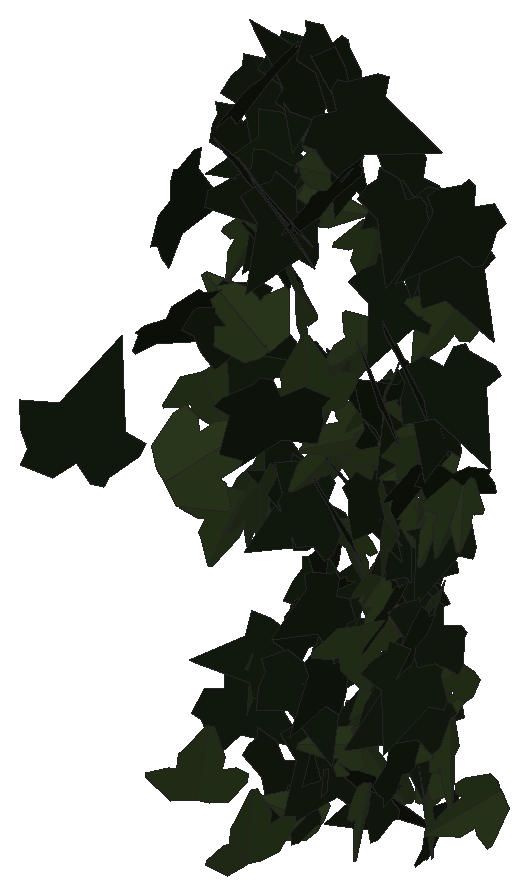
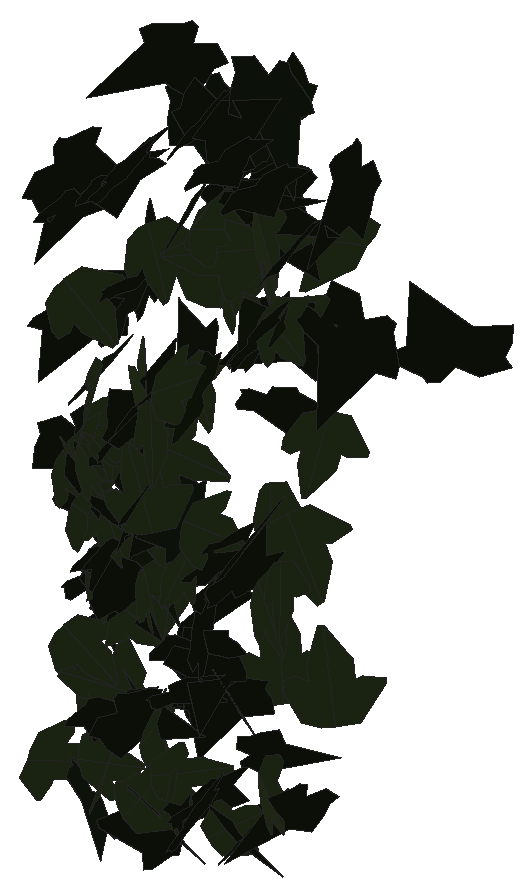
# SketchUp Ruby script. Lengths in inches.
U = 1.inch
M = Sketchup.active_model
def pt(a) = Geom::Point3d.new(a.map { |v| v * U })
def face(e, loops, mat)
  f = e.add_face(loops[0].map { |a| pt(a) })
  loops[1..].each { |l| e.add_face(l.map { |a| pt(a) }).erase! }
  f.material = f.back_material = mat if mat
  f
end
# faces: each face lists its corners as indices into pts; further lists are holes
def faces(e, pts, list, mat = nil) = list.each { |f| face(e, (f[0].is_a?(Array) ? f : [f]).map { |l| l.map { |i| pts[i] } }, mat) }
# xy, xz, yz: faces in a plane at the given z, y or x. An outline is a flat list of corners, or four numbers for a rectangle; further outlines are holes
def ring(l) = l.size == 4 ? [[l[0], l[1]], [l[2], l[1]], [l[2], l[3]], [l[0], l[3]]] : l.each_slice(2).to_a
def flat(e, list, mat, &to3) = list.each { |f| face(e, (f[0].is_a?(Array) ? f : [f]).map { |l| ring(l).map { |u, v| to3.(u, v) } }, mat) }
def xy(e, z, list, mat = nil) = flat(e, list, mat) { |x, y| [x, y, z] }
def xz(e, y, list, mat = nil) = flat(e, list, mat) { |x, z| [x, y, z] }
def yz(e, x, list, mat = nil) = flat(e, list, mat) { |y, z| [x, y, z] }
def lines(e, pts, list) = list.each { |a, b| e.add_line(pt(pts[a]), pt(pts[b])) }
# prism: a flat outline (further loops are holes) pulled along v
def prism(e, loops, v, mat = nil)
  f = face(e, loops, mat); d = Geom::Vector3d.new(v.map { |x| x * U })
  f.pushpull(f.normal.samedirection?(d) ? d.length : -d.length)
end
def box(e, o, s, mat = nil) = prism(e, [[o, [o[0] + s[0], o[1], o[2]], [o[0] + s[0], o[1] + s[1], o[2]], [o[0], o[1] + s[1], o[2]]]], [0, 0, s[2]], mat)
def at(x, y, z, deg = 0) = Geom::Transformation.translation(pt([x, y, z])) * Geom::Transformation.rotation(ORIGIN, Z_AXIS, deg.degrees)
def axes(o, x, y, z) = Geom::Transformation.new([*x, 0, *y, 0, *z, 0, *pt(o).to_a, 1])
def part(name) = M.definitions.add(name)
# library, detail: a bought-in or finely detailed component or shape, given as its bounding box
def library(name, o, s) = part(name).tap { |d| box(d.entities, o, s) }
def detail(e, o, s) = box(e.add_group.entities, o, s)
def put(e, d, t, mat = nil) = e.add_instance(d, t).tap { |i| i.material = mat if mat }
def group(e, t, mat = nil) = e.add_group.tap { |g| g.transformation = t; g.material = mat if mat }.entities
root = M.entities
M.materials.add("efeu1").color = [18, 25, 13]
M.materials.add("efeu2").color = [43, 57, 29]
c1 = part("ivyleaf_10")
p = [[0,0.5,-0.03],[-0.0625,2.02,-0.43],[-0.19,2.01,-0.46],[-0.54,1.05,-0.29],[-0.52,0.625,-0.18],[-0.83,0.76,-0.28],
  [-1.16,0.64,-0.33],[-1.15,0.33,-0.24],[-0.77,-0.39,0.02],[-0.3,-0.51,0.16],[0.04,-0.48,0.23],[-0.02,2.01,-0.4375],
  [-0.06,2.01,-0.43],[0.04,-0.49,0.23],[0.67,-0.49,0.14],[1.38,0.36,-0.2],[1.375,0.51,-0.24],[0.81,0.65,-0.19],
  [0.62,0.59,-0.15],[0.6,1.09,-0.28],[0.5,1.23,-0.31]]
faces(c1.entities,p,[[0,1,2,3,4,5,6,7,8,9,10],[11,12,0,13,14,15,16,17,18,19,20]],"efeu2")
c2 = part("ivyleaf_9")
p = [[1.54,2.16,1.25],[1.36,2.04,1.19],[-0.21,0.99,0.68],[-0.71,1.11,0.82],[-0.85,0.86,0.67],[-0.8,0.17,0.21],
  [-0.9,-0.01,0.1],[-0.67,-0.16,-0.02],[-0.08,-0.08,-0.05],[-0.03,-0.6,-0.4],[0.65,-0.88,-0.66],[0.83,-0.6,-0.49],
  [1.29,-0.42,-0.43],[1.8125,-0.07,-0.26],[1.21,0.44,0.15]]
faces(c2.entities,p,[[0,1,2,3,4,5,6,7,8,9,10,11,12,13,14]],"efeu1")
put(root,c1,axes([531.67,124.5,197.65],[0.51111,0.17788,-1.07304],[0.73605,0.81633,0.48592],[0.8008,-0.86385,0.23824]))
put(root,c2,axes([527.39,125.43,196.0625],[-0.81368,-0.12856,0.81863],[0.8051,0.14899,0.82363],[-0.19619,1.14456,-0.01526]))
put(root,c2,axes([533.48,126.2,199.56],[0.07548,0.58872,-0.9233],[-0.13977,-0.91274,-0.59341],[-1.08606,0.15838,0.0122]))
put(root,c1,axes([532.22,126.64,185.43],[-0.3475,-1.0008,-0.16593],[-0.05095,-0.15796,1.0594],[-1.01318,0.3512,0.00364]))
put(root,c1,axes([529.72,127.6,186.04],[-0.77998,-0.69849,0.07567],[0.05931,0.04719,1.04701],[-0.70006,0.78222,0.0044]))
put(root,c2,axes([533.3,128.66,195.09],[0.69791,-0.24708,-0.62973],[0.62363,-0.11557,0.73649],[-0.2621,-0.93289,0.07555]))
put(root,c1,axes([532.47,128.77,198.07],[-0.705,-0.83813,-0.16697],[-0.1081,-0.12726,1.09521],[-0.84774,0.71324,-0.00079]))
put(root,c2,axes([530.03,129.12,203.81],[0.57878,-0.62248,0.69314],[0.53625,-0.44467,-0.84712],[0.76181,0.78593,0.06969]))
put(root,c2,axes([531.34,129.53,202.91],[-0.25695,-0.80421,0.44674],[-0.15046,-0.42086,-0.84415],[0.90758,-0.29745,-0.01347]))
put(root,c2,axes([530.54,129.21,203.48],[0.56679,-0.62146,0.50238],[0.33472,-0.37466,-0.8411],[0.72565,0.65824,-0.00442]))
put(root,c2,axes([528.23,128.375,202.71],[0.03539,0.10523,-1.08229],[-0.74277,0.79321,0.05283],[0.79418,0.73717,0.09764]))
put(root,c2,axes([533.78,130.09,198.03],[-0.08215,-0.25819,0.96773],[0.28098,-0.93793,-0.22639],[0.96136,0.25207,0.14886]))
put(root,c2,axes([532.42,129.54,203.96],[-0.33089,0.95802,-0.29231],[0.08395,-0.28024,-1.01348],[-0.99809,-0.34117,0.01166]))
put(root,c2,axes([527.61,129,198.71],[0.38203,0.98395,0.23303],[0.0845,0.21717,-1.05551],[-1.00763,0.39127,-0.00016]))
put(root,c2,axes([534.6875,130.42,190.02],[-0.37882,-0.71589,0.04601],[-0.01389,-0.0447,-0.80989],[0.71723,-0.37898,0.00862]))
put(root,c1,axes([529.51,130.28,198.34],[0.62928,0.4348,0.68302],[-0.59696,-0.33525,0.76342],[0.54699,-0.86609,0.04739]))
put(root,c1,axes([528.6,130.57,192.83],[-0.53811,-0.78375,0.34572],[-0.18084,-0.29513,-0.95054],[0.8373,-0.56743,0.01689]))
put(root,c2,axes([528.52,130.05,198.85],[0.10065,-0.13279,-0.94088],[0.38967,0.86869,-0.08091],[0.86663,-0.37518,0.14566]))
put(root,c1,axes([532.88,130.43,190.41],[-0.58926,-0.74693,-0.07449],[0.03867,0.06436,-0.95133],[0.74963,-0.59045,-0.00947]))
put(root,c2,axes([534.42,131.3,188.79],[-0.54804,-0.56212,0.5967],[-0.32904,-0.50657,-0.77943],[0.75084,-0.63229,0.09397]))
put(root,c1,axes([527.66,130.48,196.2],[-0.5787,-0.66826,-0.24815],[0.18638,0.16666,-0.88348],[0.68805,-0.6072,0.03061]))
put(root,c1,axes([532.57,130.9,185.26],[0.55846,-0.42346,0.37129],[0.28299,-0.24108,-0.70061],[0.48692,0.62579,-0.01865]))
put(root,c2,axes([529.92,130.99,202.37],[-0.2292,-0.2432,-0.87783],[-0.58227,-0.65698,0.33405],[-0.70049,0.62569,0.00955]))
put(root,c1,axes([529.35,130.52,193.49],[0.03346,-0.86339,-0.31702],[-0.01158,0.31681,-0.86404],[0.91968,0.0354,0.00065]))
put(root,c1,axes([530.2,131.06,199.33],[-0.33063,0.05857,0.92811],[0.85559,-0.36682,0.32794],[0.3644,0.91441,0.07211]))
put(root,c2,axes([534.49,130.56,190.6],[-0.47537,0.61769,0.22037],[-0.15614,0.15775,-0.77898],[-0.63697,-0.49965,0.02649]))
put(root,c2,axes([529.52,130.44,205.88],[-0.29364,1.0553,-0.04247],[0.0081,-0.04183,-1.09538],[-1.05612,-0.29373,0.00341]))
put(root,c2,axes([534.21,130.42,186.84],[-0.59121,0.24381,-0.4919],[-0.45428,0.18867,0.6395],[0.30828,0.74558,-0.00097]))
put(root,c2,axes([532.25,130.35,205.9],[0.30595,-0.14445,-0.95844],[0.09276,1.0048,-0.12182],[0.96481,-0.05079,0.31564]))
put(root,c1,axes([530.31,131.38,183.7],[0.17455,0.31577,0.68802],[-0.3241,-0.60692,0.36077],[0.68414,-0.36808,-0.00463]))
put(root,c1,axes([533.51,130.57,194.07],[0.40596,-0.51903,-0.73941],[-0.12183,0.77177,-0.60864],[0.89514,0.34043,0.2525]))
put(root,c2,axes([530.91,131.62,188.28],[0.0045,-0.01792,-0.78132],[0.45338,-0.63636,0.0172],[-0.63658,-0.45335,0.00673]))
put(root,c2,axes([533.29,131,190.98],[-0.49151,0.63087,-0.02799],[0.01142,-0.02658,-0.79971],[-0.63139,-0.49159,0.00733]))
put(root,c2,axes([530.84,131.78,190.26],[0.05414,-0.31171,-0.71457],[0.27075,-0.66419,0.31024],[-0.73107,-0.26906,0.06198]))
put(root,c2,axes([533.26,131.71,198.29],[0.28539,-0.58014,0.71659],[0.31114,-0.64553,-0.64653],[0.86791,0.42218,-0.00386]))
put(root,c2,axes([528.67,131.53,197.29],[-0.60229,-0.52715,-0.17902],[0.14904,0.10144,-0.80011],[0.5364,-0.62009,0.0213]))
put(root,c2,axes([533.1,131.9375,202.81],[-0.07263,-0.84154,0.32876],[0.01939,-0.33119,-0.84349],[0.90327,-0.06056,0.04454]))
put(root,c1,axes([528.91,131.49,201.11],[0.52568,-0.78921,-0.03559],[-0.01224,0.03461,-0.94822],[0.78992,0.52575,0.00899]))
put(root,c1,axes([531.1,131.61,197.07],[0.07114,-0.80053,0.19116],[0.03911,-0.18837,-0.8034],[0.82211,0.07824,0.02168]))
put(root,c2,axes([530.12,131.53,188.04],[-0.22868,-0.69251,-0.56329],[0.13918,0.54671,-0.72863],[0.88176,-0.2659,-0.03108]))
put(root,c2,axes([530.39,131.47,184.09],[-0.62627,0.30407,0.34465],[-0.31126,0.14801,-0.69618],[-0.33817,-0.69935,0.00251]))
put(root,c2,axes([528.9,132.12,184.48],[0.02065,-0.79307,0.43311],[0.10958,-0.42782,-0.78862],[0.89696,0.07053,0.08637]))
put(root,c2,axes([529.375,132.05,202.91],[-0.56755,-0.19683,0.57563],[-0.46781,-0.36205,-0.58505],[0.38891,-0.72276,0.1363]))
put(root,c2,axes([534.15,132.14,190.39],[-0.38078,-0.68788,0.31013],[-0.14989,-0.27151,-0.78624],[0.73952,-0.40922,0.00033]))
put(root,c1,axes([528.54,131.96,202.59],[0.28329,-0.82773,0.04286],[0.01181,-0.04126,-0.87487],[0.82876,0.28352,-0.00218]))
put(root,c2,axes([529.89,132.58,192.39],[-0.45454,-0.53355,0.66094],[-0.32369,-0.58426,-0.69425],[0.78533,-0.54963,0.09639]))
put(root,c2,axes([530.29,132.55,185.09],[-0.31722,-0.76634,0.45104],[-0.16937,-0.41804,-0.8294],[0.87294,-0.35959,0.00298]))
put(root,c2,axes([532.61,132.46,199.83],[-0.27111,-0.78331,0.29293],[-0.02178,-0.30122,-0.82563],[0.836,-0.26187,0.07348]))
put(root,c2,axes([533.71,132.4375,196.47],[-0.0157,-0.7081,0.43658],[0.11215,-0.43447,-0.70065],[0.82428,0.04563,0.10365]))
put(root,c1,axes([534.27,132.23,187.07],[0.61305,-0.31717,0.59025],[0.52859,-0.26275,-0.6902],[0.4118,0.80943,0.00724]))
put(root,c1,axes([527.84,132.36,200.11],[-0.05149,-0.67931,0.45198],[0.01496,-0.45359,-0.68002],[0.8158,-0.03456,0.04099]))
put(root,c1,axes([532.07,132.48,196.3],[0.17153,-0.50151,-0.71944],[0.27373,-0.66584,0.5294],[-0.83318,-0.322,0.02581]))
put(root,c2,axes([533.08,132.35,202.65],[-0.11703,-0.85653,-0.12764],[0.00054,0.12873,-0.86433],[0.86599,-0.11583,-0.01671]))
put(root,c1,axes([531.46,132.38,195.1],[-0.20095,-0.21076,0.84653],[-0.64041,-0.55424,-0.29001],[0.59237,-0.67068,-0.02636]))
put(root,c2,axes([530.45,132.19,197.02],[0.68532,-0.63545,0.17635],[0.12994,-0.11923,-0.93459],[0.64654,0.69753,0.0009]))
put(root,c2,axes([533.7,132,195.09],[-0.31589,0.83525,-0.38794],[0.1227,-0.3683,-0.89287],[-0.91273,-0.33859,0.01424]))
put(root,c2,axes([528.125,132.58,199.48],[0.07607,-0.58224,0.6331],[0.39217,-0.54218,-0.54575],[0.76552,0.33562,0.21667]))
put(root,c2,axes([529.4,132.67,192.11],[0.23944,-0.8888,-0.18002],[0.09505,-0.16057,0.91918],[-0.90185,-0.2529,0.04908]))
put(root,c2,axes([529.27,132.49,188.72],[-0.53436,-0.0974,-0.54403],[0.55223,-0.12473,-0.52008],[-0.02237,-0.7523,0.15667]))
put(root,c1,axes([531.11,132.63,185.65],[-0.0512,0.14739,0.80501],[-0.39738,-0.70959,0.10465],[0.71544,-0.38358,0.11574]))
put(root,c2,axes([534.32,132.11,198.13],[-0.06021,-0.71576,-0.66616],[0.11222,0.65795,-0.71709],[0.97134,-0.12038,0.04156]))
put(root,c2,axes([528.33,132.53,187.23],[-0.47983,-0.05752,0.58833],[-0.57054,-0.15321,-0.4803],[0.15468,-0.74357,0.05346]))
put(root,c2,axes([530.1,132.24,204.76],[0.14325,-0.09433,0.92606],[-0.84117,0.38814,0.16965],[-0.39864,-0.85291,-0.02521]))
put(root,c2,axes([534.56,132.9,202.6875],[0.01218,-0.06148,-0.96523],[0.26498,-0.92816,0.06246],[-0.93018,-0.26521,0.00516]))
put(root,c1,axes([530.09,132.72,202.2],[-0.32762,0.44575,0.65062],[0.13261,-0.66336,0.52125],[0.77744,0.301,0.18526]))
put(root,c1,axes([533.44,131.71,187],[-0.0902,-0.51212,0.82096],[0.14087,0.80878,0.52001],[-0.95729,0.16728,-0.00083]))
put(root,c1,axes([533.25,132.24,195.49],[-0.3719,-0.78703,-0.0816],[0.0259,0.078,-0.87041],[0.79082,-0.37267,-0.00986]))
put(root,c2,axes([532.74,133.03,202.92],[-0.32456,-0.57892,0.63941],[-0.17061,-0.62659,-0.65392],[0.84551,-0.34867,0.1135]))
put(root,c1,axes([529.32,131.93,201.54],[-0.13811,-0.08684,-0.97194],[0.91387,0.33267,-0.15958],[0.34214,-0.92362,0.03391]))
put(root,c1,axes([530.89,132.98,197.33],[-0.04742,-0.09294,0.88427],[0.14386,-0.87466,-0.08422],[0.87743,0.13839,0.06159]))
put(root,c1,axes([533.74,132.41,190.9],[0.20839,-0.7691,-0.01612],[-0.00031,0.01662,-0.79682],[0.76927,0.20835,0.00405]))
put(root,c2,axes([532.1,132.78,195.57],[0.24145,0.25043,0.83541],[-0.55266,-0.62664,0.34758],[0.67468,-0.60293,-0.01426]))
put(root,c2,axes([534.4,132.24,201.5],[0.17308,-0.67643,-0.52752],[-0.06629,0.52599,-0.69622],[0.85524,0.17766,0.05279]))
put(root,c2,axes([527.08,132.72,202.65],[0.18818,-0.82673,0.10934],[0.01831,-0.10797,-0.84786],[0.83373,0.18897,-0.00606]))
put(root,c2,axes([531.82,132.26,193.78],[0.37262,-0.72687,-0.4985],[-0.23032,0.44211,-0.81681],[0.85076,0.43805,-0.0028]))
put(root,c2,axes([528.05,132.81,204.29],[-0.2236,-0.8336,0.01086],[-0.00188,-0.01074,-0.86307],[0.83367,-0.22361,0.00097]))
put(root,c1,axes([533.28,132.52,185.28],[-0.39217,0.76754,-0.43408],[0.19469,-0.38798,-0.86192],[-0.86002,-0.43783,0.00282]))
put(root,c1,axes([531.37,133.01,186.91],[-0.17903,0.14378,0.92007],[0.44271,-0.81113,0.2129],[0.81928,0.46972,0.08601]))
put(root,c1,axes([531.74,132.52,201.28],[-0.30172,-0.79982,0.13698],[-0.04066,-0.13106,-0.8548],[0.81045,-0.30434,0.00811]))
put(root,c1,axes([529.61,133.02,202.53],[-0.04907,-0.27072,0.80584],[0.13534,-0.79938,-0.26031],[0.83926,0.11308,0.08909]))
put(root,c2,axes([532.18,132.42,184.41],[-0.68526,0.30854,0.21566],[-0.20594,0.06766,-0.75119],[-0.3151,-0.7152,0.02196]))
put(root,c1,axes([527.62,132.3125,192.62],[0.00733,-0.75862,-0.2512],[-0.01029,0.2511,-0.75862],[0.79906,0.01019,-0.00746]))
put(root,c2,axes([527.14,132.03,186.09],[0.32576,-0.40309,-0.77176],[-0.04943,0.81412,-0.44608],[0.86928,0.19735,0.26385]))
put(root,c2,axes([530.53,132.53,193.46],[0.66091,-0.44203,0.28266],[0.23728,-0.15365,-0.7951],[0.46796,0.70221,0.00395]))
put(root,c1,axes([530.85,132.44,191.96],[-0.69029,0.25831,-0.25408],[0.21954,-0.13673,-0.73546],[-0.28825,-0.72275,0.04832]))
put(root,c1,axes([531.76,132.63,191.125],[0.12982,-0.84322,0.02575],[0.00133,-0.02585,-0.85315],[0.84361,0.1298,-0.00262]))
put(root,c1,axes([529.76,133.11,193.73],[-0.0711,-0.45967,0.71018],[-0.04085,-0.70999,-0.46363],[0.84497,-0.073,0.03734]))
put(root,c1,axes([527.74,132.82,192.21],[0.15395,-0.87739,0.21557],[0.0745,-0.20561,-0.89003],[0.90041,0.16702,0.03679]))
put(root,c1,axes([534.91,133.11,185.07],[0.16818,0.25385,-0.85963],[-0.51535,-0.68821,-0.30405],[-0.73335,0.54185,0.01654]))
put(root,c1,axes([534.11,132.93,194],[-0.04553,-0.77495,0.37342],[0.09438,-0.37618,-0.76918],[0.85503,0.00026,0.10479]))
put(root,c1,axes([534.11,132.8,188.76],[-0.44427,-0.33049,0.57072],[-0.44666,-0.35551,-0.55356],[0.48522,-0.62985,0.01298]))
put(root,c1,axes([532.68,132.93,195.66],[0.14959,0.15587,-0.75993],[-0.65901,-0.38277,-0.20823],[-0.40926,0.67332,0.05754]))
put(root,c2,axes([532.27,133.29,195.73],[-0.11072,-0.70925,0.54184],[-0.07656,-0.53643,-0.71782],[0.88925,-0.13449,0.00567]))
put(root,c2,axes([530.11,133.27,202.74],[0.08457,-0.67732,0.57446],[0.04194,-0.57337,-0.68221],[0.88714,0.09167,-0.02251]))
put(root,c2,axes([532.8,132.89,191.93],[-0.15177,-0.76253,-0.2035],[0.07066,0.19327,-0.77689],[0.78605,-0.16461,0.03054]))
put(root,c1,axes([532.03,132.91,190.23],[0.42292,0.47298,-0.45949],[-0.29748,-0.35032,-0.63441],[-0.58851,0.51698,-0.00952]))
put(root,c2,axes([529.62,133.22,189.97],[0.0456,0.1184,0.86302],[-0.16992,-0.8464,0.1251],[0.85438,-0.17465,-0.02118]))
put(root,c2,axes([529.72,133.12,205.77],[0.1632,-0.83329,0.14888],[0.00332,-0.15099,-0.84874],[0.84648,0.16125,-0.02538]))
put(root,c1,axes([534.27,132.82,194.22],[0.75457,-0.16498,0.20367],[0.20083,-0.03491,-0.77235],[0.16842,0.78079,0.00851]))
put(root,c2,axes([528.92,132.67,192.02],[-0.40967,-0.73337,0.39954],[0.19291,0.34989,0.84003],[-0.81256,0.45281,-0.00201]))
put(root,c1,axes([532.09,132.75,184.53],[-0.76383,0.09156,-0.56397],[-0.5609,0.05912,0.76927],[0.1088,0.94763,0.00649]))
put(root,c2,axes([530.09,132.94,190.11],[-0.39628,-0.67108,-0.32278],[0.14329,0.29009,-0.77904],[0.73076,-0.4208,-0.02228]))
put(root,c2,axes([534.21,132.59,194.77],[0.20083,0.62114,-0.45863],[-0.23501,-0.40223,-0.64766],[-0.73548,0.29813,0.08172]))
put(root,c1,axes([533.29,132.99,195.15],[0.44754,0.23412,-0.66488],[-0.59627,-0.2943,-0.50499],[-0.37595,0.74548,0.00945]))
put(root,c2,axes([531,132.71,184.19],[0.60429,-0.22546,0.53768],[0.51303,-0.1623,-0.64464],[0.27702,0.79242,0.02095]))
put(root,c2,axes([529.87,132.37,189.72],[0.20499,0.74337,-0.04594],[-0.01374,-0.04387,-0.77111],[-0.74466,0.20544,0.00158]))
put(root,c2,axes([533.67,133.05,193.1],[-0.75378,-0.27842,-0.31916],[0.30139,0.10515,-0.80354],[0.29757,-0.81178,0.00538]))
put(root,c2,axes([532.15,133.3,187.43],[-0.02005,-0.14138,-0.81916],[-0.1538,-0.80463,0.14263],[-0.81692,0.15495,-0.00675]))
put(root,c1,axes([533.0625,132.91,193.02],[-0.65212,-0.34574,0.33267],[-0.24422,-0.24399,-0.73232],[0.41299,-0.69022,0.09224]))
put(root,c2,axes([532.56,133.01,187.47],[-0.24837,-0.83847,-0.37533],[0.1154,0.35724,-0.87444],[0.91136,-0.27374,0.00844]))
put(root,c2,axes([529.79,133.5625,185.06],[-0.13183,-0.58996,0.70305],[-0.10208,-0.69643,-0.60355],[0.91209,-0.16322,0.03407]))
put(root,c1,axes([533.77,133.2,199.27],[-0.43282,-0.59665,0.54528],[-0.23122,-0.50129,-0.73205],[0.7745,-0.48308,0.08618]))
put(root,c1,axes([531.54,132.73,196.17],[0.01117,-0.84532,-0.23235],[-0.00693,0.23227,-0.84539],[0.87664,0.01261,-0.00373]))
put(root,c1,axes([527.4,133.2,186.92],[0.38205,-0.74233,0.4175],[0.24249,-0.34383,-0.83325],[0.81643,0.4495,0.05212]))
put(root,c1,axes([533.3125,133.24,194.6875],[0.23016,-0.74794,0.4424],[0.15445,-0.41515,-0.78224],[0.85515,0.27629,0.02221]))
put(root,c2,axes([530.375,133.37,188.75],[-0.49451,-0.55629,0.24804],[-0.09126,-0.24822,-0.73863],[0.6022,-0.49442,0.09174]))
put(root,c2,axes([532.96,132.84,191.12],[0.04245,0.13758,-0.7754],[-0.64819,-0.4349,-0.11265],[-0.44724,0.64336,0.08967]))
put(root,c2,axes([527.74,133.5,200.07],[-0.13678,-0.67304,0.51776],[-0.1185,-0.50418,-0.68668],[0.84084,-0.18054,-0.01255]))
put(root,c2,axes([528.86,133.32,205],[-0.19398,-0.84548,0.06048],[-0.01348,-0.05896,-0.86745],[0.84754,-0.19444,0.00005]))
put(root,c2,axes([532.6,132.86,192.17],[0.19916,-0.65973,-0.36905],[-0.11269,0.35147,-0.68911],[0.74749,0.22876,-0.00556]))
put(root,c1,axes([533.42,132.85,185.45],[-0.13166,0.03384,-0.79601],[-0.78066,0.15573,0.13574],[0.15919,0.79165,0.00733]))
put(root,c2,axes([533.9,132.35,184.04],[-0.21414,0.63683,0.54638],[-0.16912,0.51956,-0.67186],[-0.82188,-0.27284,-0.00411]))
put(root,c1,axes([531.53,132.95,193.4375],[-0.81821,-0.40103,0.29579],[0.27423,0.11244,0.91102],[-0.41608,0.86274,0.01876]))
put(root,c1,axes([533.49,132.72,196.66],[-0.47756,0.63249,0.08716],[-0.05887,0.06476,-0.79249],[-0.63575,-0.48111,0.00791]))
put(root,c1,axes([533.34,133.42,193.09],[-0.10635,-0.53862,0.60657],[0.18475,-0.61177,-0.51084],[0.78987,0.07057,0.20116]))
